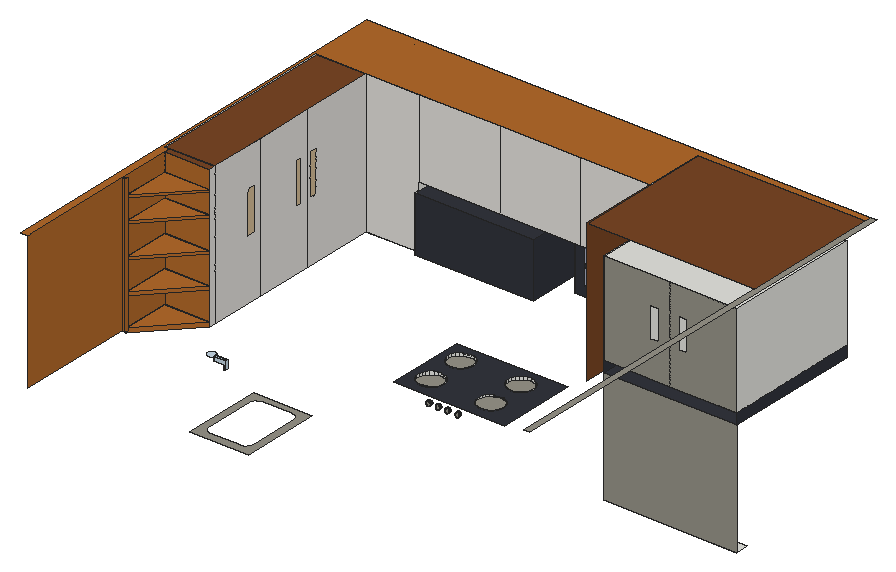
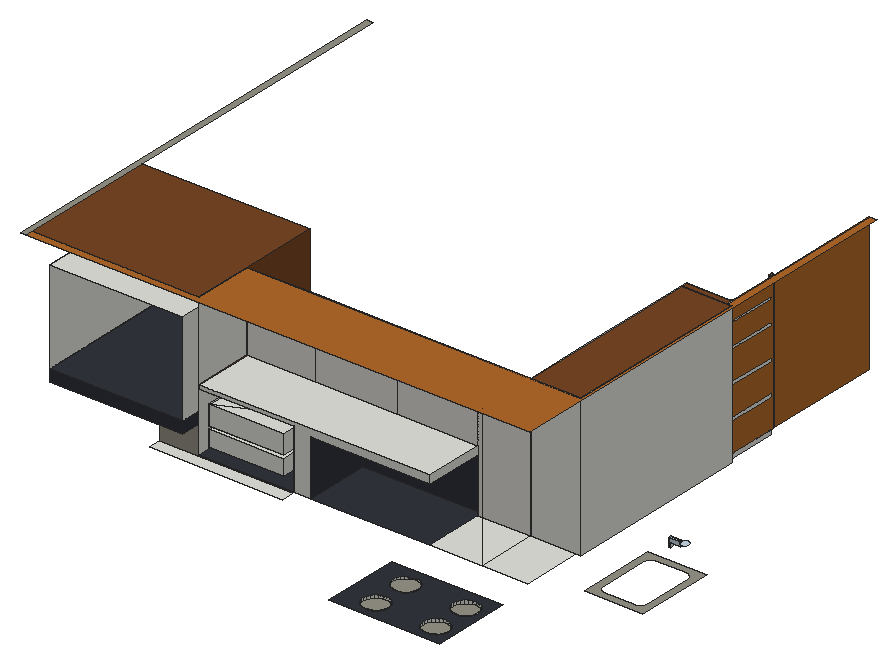
# SketchUp Ruby script. Lengths in inches.
U = 1.inch
M = Sketchup.active_model
def pt(a) = Geom::Point3d.new(a.map { |v| v * U })
def face(e, loops, mat)
  f = e.add_face(loops[0].map { |a| pt(a) })
  loops[1..].each { |l| e.add_face(l.map { |a| pt(a) }).erase! }
  f.material = f.back_material = mat if mat
  f
end
# faces: each face lists its corners as indices into pts; further lists are holes
def faces(e, pts, list, mat = nil) = list.each { |f| face(e, (f[0].is_a?(Array) ? f : [f]).map { |l| l.map { |i| pts[i] } }, mat) }
# xy, xz, yz: faces in a plane at the given z, y or x. An outline is a flat list of corners, or four numbers for a rectangle; further outlines are holes
def ring(l) = l.size == 4 ? [[l[0], l[1]], [l[2], l[1]], [l[2], l[3]], [l[0], l[3]]] : l.each_slice(2).to_a
def flat(e, list, mat, &to3) = list.each { |f| face(e, (f[0].is_a?(Array) ? f : [f]).map { |l| ring(l).map { |u, v| to3.(u, v) } }, mat) }
def xy(e, z, list, mat = nil) = flat(e, list, mat) { |x, y| [x, y, z] }
def xz(e, y, list, mat = nil) = flat(e, list, mat) { |x, z| [x, y, z] }
def yz(e, x, list, mat = nil) = flat(e, list, mat) { |y, z| [x, y, z] }
def lines(e, pts, list) = list.each { |a, b| e.add_line(pt(pts[a]), pt(pts[b])) }
# prism: a flat outline (further loops are holes) pulled along v
def prism(e, loops, v, mat = nil)
  f = face(e, loops, mat); d = Geom::Vector3d.new(v.map { |x| x * U })
  f.pushpull(f.normal.samedirection?(d) ? d.length : -d.length)
end
def box(e, o, s, mat = nil) = prism(e, [[o, [o[0] + s[0], o[1], o[2]], [o[0] + s[0], o[1] + s[1], o[2]], [o[0], o[1] + s[1], o[2]]]], [0, 0, s[2]], mat)
def at(x, y, z, deg = 0) = Geom::Transformation.translation(pt([x, y, z])) * Geom::Transformation.rotation(ORIGIN, Z_AXIS, deg.degrees)
def axes(o, x, y, z) = Geom::Transformation.new([*x, 0, *y, 0, *z, 0, *pt(o).to_a, 1])
def part(name) = M.definitions.add(name)
# library, detail: a bought-in or finely detailed component or shape, given as its bounding box
def library(name, o, s) = part(name).tap { |d| box(d.entities, o, s) }
def detail(e, o, s) = box(e.add_group.entities, o, s)
def put(e, d, t, mat = nil) = e.add_instance(d, t).tap { |i| i.material = mat if mat }
def group(e, t, mat = nil) = e.add_group.tap { |g| g.transformation = t; g.material = mat if mat }.entities
root = M.entities
M.materials.add("[Formica Beige]").color = [211, 187, 149]
M.materials.add("[Formica Graystone]").color = [149, 146, 135]
M.materials.add("[Formica Laminate Dark]").color = [50, 53, 60]
M.materials.add("[Terrazzo Light Blue]").color = [196, 214, 227]
M.materials.add("[Terrazzo Tile Accent]").color = [224, 221, 217]
M.materials.add("[Translucent Glass Sky Reflection]").color = [126, 138, 183]
M.materials["[Translucent Glass Sky Reflection]"].alpha = 0.52
M.materials.add("[Wood Bamboo]").color = [177, 105, 43]
M.materials.add("[Wood Veneer 01]").color = [120, 70, 37]
xy(root,44.875,[[[7.92,55.33,25.99,79.71],[12.63,57.43,12.29,57.45,11.96,57.52,11.63,57.625,11.33,57.78,11.04,57.97,10.78,58.19,10.56,58.45,10.37,58.73,10.22,59.04,10.11,59.36,10.04,59.7,10.02,60.04,10.02,75.53,10.04,75.8,10.09,76.07,10.18,76.33,10.3,76.57,10.45,76.8,10.63,77,10.84,77.18,11.0625,77.33,11.31,77.45,11.57,77.54,11.83,77.6,12.11,77.61,21.58,77.61,21.89,77.59,22.18,77.53,22.47,77.4375,22.74,77.3,22.99,77.14,23.22,76.9375,23.42,76.71,23.58,76.46,23.72,76.1875,23.8125,75.9,23.87,75.61,23.89,75.31,23.89,59.85,23.87,59.54,23.81,59.23,23.71,58.93,23.57,58.64,23.39,58.375,23.18,58.14,22.94,57.93,22.68,57.75,22.39,57.61,22.09,57.51,21.78,57.45,21.47,57.43]]],"[Formica Graystone]")
xy(root,46.625,[[40.04,104,41.05,104.13,41.98,104.52,42.78,105.13,43.4,105.93,43.79,106.87,43.92,107.87,43.79,108.875,43.4,109.81,42.78,110.61,41.98,111.23,41.05,111.61,40.04,111.75,39.04,111.61,38.11,111.23,37.3,110.61,36.6875,109.81,36.3,108.875,36.17,107.87,36.3,106.87,36.6875,105.93,37.3,105.13,38.11,104.52,39.04,104.13]],"[Formica Graystone]")
xy(root,46.64,[[108.5,88.5625,149.5,92.5]])
xy(root,46.6875,[[39.92,115.43,40.92,115.57,41.86,115.95,42.66,116.57,43.27,117.37,43.66,118.31,43.79,119.31,43.66,120.3125,43.27,121.25,42.66,122.05,41.86,122.66,40.92,123.05,39.92,123.18,38.92,123.05,37.98,122.66,37.18,122.05,36.5625,121.25,36.17,120.3125,36.04,119.31,36.17,118.31,36.5625,117.37,37.18,116.57,37.98,115.95,38.92,115.57],[58.48,115.43,59.48,115.57,60.42,115.95,61.22,116.57,61.84,117.37,62.22,118.31,62.36,119.31,62.22,120.3125,61.84,121.25,61.22,122.05,60.42,122.66,59.48,123.05,58.48,123.18,57.48,123.05,56.54,122.66,55.74,122.05,55.125,121.25,54.74,120.3125,54.61,119.31,54.74,118.31,55.125,117.37,55.74,116.57,56.54,115.95,57.48,115.57]],"[Formica Graystone]")
xy(root,47.0625,[[58.48,104,59.48,104.13,60.42,104.52,61.22,105.13,61.84,105.93,62.22,106.87,62.36,107.87,62.22,108.875,61.84,109.81,61.22,110.61,60.42,111.23,59.48,111.61,58.48,111.75,57.48,111.61,56.54,111.23,55.74,110.61,55.125,109.81,54.74,108.875,54.61,107.87,54.74,106.87,55.125,105.93,55.74,105.13,56.54,104.52,57.48,104.13]],"[Formica Graystone]")
xy(root,47.5,[[[34.11,101.1,68.05,125.35],[39.92,115.43,38.92,115.57,37.98,115.95,37.18,116.57,36.5625,117.37,36.17,118.31,36.04,119.31,36.17,120.3125,36.5625,121.25,37.18,122.05,37.98,122.66,38.92,123.05,39.92,123.18,40.92,123.05,41.86,122.66,42.66,122.05,43.27,121.25,43.66,120.3125,43.79,119.31,43.66,118.31,43.27,117.37,42.66,116.57,41.86,115.95,40.92,115.57],[58.48,115.43,57.48,115.57,56.54,115.95,55.74,116.57,55.125,117.37,54.74,118.31,54.61,119.31,54.74,120.3125,55.125,121.25,55.74,122.05,56.54,122.66,57.48,123.05,58.48,123.18,59.48,123.05,60.42,122.66,61.22,122.05,61.84,121.25,62.22,120.3125,62.36,119.31,62.22,118.31,61.84,117.37,61.22,116.57,60.42,115.95,59.48,115.57],[58.48,104,57.48,104.13,56.54,104.52,55.74,105.13,55.125,105.93,54.74,106.87,54.61,107.87,54.74,108.875,55.125,109.81,55.74,110.61,56.54,111.23,57.48,111.61,58.48,111.75,59.48,111.61,60.42,111.23,61.22,110.61,61.84,109.81,62.22,108.875,62.36,107.87,62.22,106.87,61.84,105.93,61.22,105.13,60.42,104.52,59.48,104.13],[40.04,104,39.04,104.13,38.11,104.52,37.3,105.13,36.6875,105.93,36.3,106.87,36.17,107.87,36.3,108.875,36.6875,109.81,37.3,110.61,38.11,111.23,39.04,111.61,40.04,111.75,41.05,111.61,41.98,111.23,42.78,110.61,43.4,109.81,43.79,108.875,43.92,107.87,43.79,106.87,43.4,105.93,42.78,105.13,41.98,104.52,41.05,104.13]]],"[Formica Laminate Dark]")
xy(root,57.375,[[9.09,66.7,9.81,67.6]])
xy(root,58.5625,[[6.04,66.7,6.16,66.99,6.2,67.29,6.16,67.6,9.09,67.6,9.09,66.7]])
xy(root,59.875,[[6.04,66.7,6.16,66.99,6.2,67.29,6.16,67.6,6.04,67.6]])
xy(root,59.875,[[5.01,66.11,5.32,66.15,5.61,66.27,5.85,66.45,6.04,66.7,6.04,67.6,6.16,67.6,6.04,67.89,5.85,68.13,5.61,68.32,5.32,68.44,5.01,68.48,4.71,68.44,4.42,68.32,4.17,68.13,3.99,67.89,3.87,67.6,3.83,67.29,3.87,66.99,3.99,66.7,4.17,66.45,4.42,66.27,4.71,66.15],[6.04,66.7,9.81,66.7,9.81,67.6,6.16,67.6,6.2,67.29,6.16,66.99]],"[Terrazzo Light Blue]")
xy(root,77.75,[[0.9375,54.54,2.25,112.625],[2.25,112.625,16.25,131.0625],[16.25,112.625,32.46,131.0625]])
xy(root,77.75,[[32.46,111.0625,68.96,131.0625],[74.1875,120.3125,103.5,131.0625]],"[Formica Laminate Dark]")
xy(root,77.75,[[2.25,37.75,2.25,52.57,16.25,52.57],[2.25,52.57,16.25,54.54],[2.25,54.54,16.25,112.625]],"[Wood Bamboo]")
xy(root,79.12,[[2.25,36.1,3.375,36.93],[2.25,37.75,16.25,52.57,2.25,52.57]],"[Wood Bamboo]")
xy(root,80.93,[[77.37,120.3125,100.32,131.0625]])
xy(root,81.6875,[[108.5,88.5625,149.5,131.0625]],"[Formica Laminate Dark]")
xy(root,85.21,[[108.5,88.5625,149.5,131.0625]],"[Formica Laminate Dark]")
xy(root,85.84,[[77.37,120.3125,100.32,131.0625]])
xy(root,86.81,[[77.37,120.3125,100.32,131.0625]])
xy(root,88,[[2.25,37.75,2.25,52.57,16.25,52.57]],"[Wood Bamboo]")
xy(root,89.06,[[2.25,37.75,16.25,52.57,2.25,52.57]],"[Wood Bamboo]")
xy(root,92.68,[[77.37,120.3125,100.32,131.0625,100.32,120.3125],[77.37,120.3125,77.37,131.0625,100.32,131.0625]])
xy(root,94.62,[[32.46,111.0625,68.96,131.0625]],"[Formica Laminate Dark]")
xy(root,95.86,[[74.1875,120.3125,103.5,131.0625]])
xy(root,96.97,[[32.46,112.625,103.5,131.0625]])
xy(root,97.9,[[2.25,37.75,2.25,52.57,16.25,52.57]],"[Wood Bamboo]")
xy(root,98.72,[[2.25,37.75,16.25,52.57,2.25,52.57]],"[Wood Bamboo]")
xy(root,107.81,[[2.25,37.75,2.25,52.57,16.25,52.57]],"[Wood Bamboo]")
xy(root,108.56,[[2.25,37.75,16.25,52.57,2.25,52.57]],"[Wood Bamboo]")
xy(root,113.88,[[108.5,88.5625,149.5,131.0625]])
xy(root,115,[[2.25,37.75,2.25,52.57,16.25,52.57]],"[Wood Bamboo]")
xy(root,115.68,[[2.25,37.75,16.25,52.57,2.25,52.57]],"[Wood Bamboo]")
xy(root,121.1875,[[154.9375,0,156.6875,133.25]],"[Formica Graystone]")
xy(root,121.1875,[[0,0,2.25,0,2.25,36.1,3.375,36.1,3.375,36.93,2.25,36.93,2.25,54.54,0.9375,54.54,0.9375,112.625,103.5,112.625,103.5,131.0625,154.9375,131.0625,154.9375,133.25,0,133.25]],"[Wood Bamboo]")
xy(root,121.1875,[[2.25,52.57,16.25,54.54],[0.9375,54.54,16.25,112.625],[103.5,88.5625,154.9375,131.0625]],"[Wood Veneer 01]")
xz(root,36.1,[[2.25,79.12,3.375,121.1875]],"[Wood Bamboo]")
xz(root,36.93,[[2.25,79.12,3.375,121.1875]],"[Wood Bamboo]")
xz(root,52.57,[[2.25,77.75,16.25,79.12],[2.25,88,16.25,89.06],[2.25,97.9,16.25,98.72],[2.25,107.81,16.25,108.56],[2.25,115,16.25,115.68]])
xz(root,52.57,[[2.25,79.12,16.25,88],[2.25,89.06,16.25,97.9],[2.25,98.72,16.25,107.81],[2.25,108.56,16.25,115],[2.25,115.68,16.25,121.1875]],"[Wood Bamboo]")
xz(root,54.54,[[0.9375,77.75,2.25,121.1875],[2.25,77.75,16.25,121.1875]])
xz(root,66.7,[[9.09,57.375,9.81,57.375,9.81,59.875,6.04,59.875,6.04,58.5625,9.09,58.5625]],"[Terrazzo Light Blue]")
xz(root,67.6,[[9.09,57.375,9.09,58.5625,6.16,58.5625,6.16,59.875,9.81,59.875,9.81,57.375]],"[Terrazzo Light Blue]")
xz(root,88.5625,[[123.23,96.37,125.23,105.31],[131.86,96.37,133.86,105.31]])
xz(root,88.5625,[[108.5,46.64,149.5,81.6875],[[108.5,85.21,129,113.88],[123.23,96.37,125.23,105.31]],[[129,85.21,149.5,113.88],[131.86,96.37,133.86,105.31]]],"[Formica Graystone]")
xz(root,100.41,[[45.19,45.12,45.37,45.14,45.54,45.21,45.68,45.32,45.79,45.46,45.86,45.625,45.88,45.8,45.86,45.98,45.79,46.15,45.68,46.29,45.54,46.4,45.37,46.47,45.19,46.49,45.02,46.47,44.85,46.4,44.71,46.29,44.6,46.15,44.53,45.98,44.51,45.8,44.53,45.625,44.6,45.46,44.71,45.32,44.85,45.21,45.02,45.14],[48.01,45.12,48.18,45.14,48.35,45.21,48.49,45.32,48.6,45.46,48.67,45.625,48.69,45.8,48.67,45.98,48.6,46.15,48.49,46.29,48.35,46.4,48.18,46.47,48.01,46.49,47.83,46.47,47.66,46.4,47.52,46.29,47.41,46.15,47.34,45.98,47.32,45.8,47.34,45.625,47.41,45.46,47.52,45.32,47.66,45.21,47.83,45.14],[50.88,45.12,51.06,45.14,51.22,45.21,51.37,45.32,51.48,45.46,51.55,45.625,51.57,45.8,51.55,45.98,51.48,46.15,51.37,46.29,51.22,46.4,51.06,46.47,50.88,46.49,50.7,46.47,50.54,46.4,50.39,46.29,50.29,46.15,50.22,45.98,50.19,45.8,50.22,45.625,50.29,45.46,50.39,45.32,50.54,45.21,50.7,45.14],[54.07,45.12,54.25,45.14,54.41,45.21,54.55,45.32,54.66,45.46,54.73,45.625,54.76,45.8,54.73,45.98,54.66,46.15,54.55,46.29,54.41,46.4,54.25,46.47,54.07,46.49,53.89,46.47,53.72,46.4,53.58,46.29,53.47,46.15,53.4,45.98,53.38,45.8,53.4,45.625,53.47,45.46,53.58,45.32,53.72,45.21,53.89,45.14]],"[Formica Graystone]")
xz(root,101.1,[[45.19,45.12,45.02,45.14,44.85,45.21,44.71,45.32,44.6,45.46,44.53,45.625,44.51,45.8,44.53,45.98,44.6,46.15,44.71,46.29,44.85,46.4,45.02,46.47,45.19,46.49,45.37,46.47,45.54,46.4,45.68,46.29,45.79,46.15,45.86,45.98,45.88,45.8,45.86,45.625,45.79,45.46,45.68,45.32,45.54,45.21,45.37,45.14],[48.01,45.12,47.83,45.14,47.66,45.21,47.52,45.32,47.41,45.46,47.34,45.625,47.32,45.8,47.34,45.98,47.41,46.15,47.52,46.29,47.66,46.4,47.83,46.47,48.01,46.49,48.18,46.47,48.35,46.4,48.49,46.29,48.6,46.15,48.67,45.98,48.69,45.8,48.67,45.625,48.6,45.46,48.49,45.32,48.35,45.21,48.18,45.14],[50.88,45.12,50.7,45.14,50.54,45.21,50.39,45.32,50.29,45.46,50.22,45.625,50.19,45.8,50.22,45.98,50.29,46.15,50.39,46.29,50.54,46.4,50.7,46.47,50.88,46.49,51.06,46.47,51.22,46.4,51.37,46.29,51.48,46.15,51.55,45.98,51.57,45.8,51.55,45.625,51.48,45.46,51.37,45.32,51.22,45.21,51.06,45.14],[54.07,45.12,53.89,45.14,53.72,45.21,53.58,45.32,53.47,45.46,53.4,45.625,53.38,45.8,53.4,45.98,53.47,46.15,53.58,46.29,53.72,46.4,53.89,46.47,54.07,46.49,54.25,46.47,54.41,46.4,54.55,46.29,54.66,46.15,54.73,45.98,54.76,45.8,54.73,45.625,54.66,45.46,54.55,45.32,54.41,45.21,54.25,45.14]])
xz(root,111.0625,[[32.46,77.75,68.96,94.62]],"[Formica Laminate Dark]")
xz(root,112.625,[[0.9375,77.75,16.25,121.1875]])
xz(root,112.625,[[16.25,77.75,32.46,121.1875],[32.46,96.97,57.4375,121.1875],[57.4375,96.97,82.42,121.1875],[82.42,96.97,103.5,121.1875]],"[Terrazzo Tile Accent]")
xz(root,120.3125,[[[74.1875,77.75,103.5,95.86],[77.37,80.93,100.32,92.68]],[77.37,85.84,100.32,86.81]],"[Formica Laminate Dark]")
xz(root,120.3125,[[77.37,80.93,100.32,85.84],[77.37,86.81,100.32,92.68]],"[Translucent Glass Sky Reflection]")
xz(root,131.0625,[[68.96,77.75,74.1875,77.75,74.1875,95.86,103.5,95.86,103.5,96.97,32.46,96.97,32.46,94.62,68.96,94.62],[77.37,80.93,100.32,85.84],[77.37,86.81,100.32,92.68]])
xz(root,131.0625,[[108.5,81.6875,149.5,85.21]],"[Formica Laminate Dark]")
yz(root,0.9375,[[54.54,77.75,112.625,121.1875]])
yz(root,2.25,[[37.75,77.75,52.57,79.12],[52.57,77.75,54.54,121.1875],[37.75,88,52.57,89.06],[37.75,97.9,52.57,98.72],[37.75,107.81,52.57,108.56],
  [37.75,115,52.57,115.68]])
yz(root,2.25,[[0,79.12,36.1,121.1875],[36.93,79.12,52.57,79.12,52.57,88,37.75,88,37.75,89.06,52.57,89.06,52.57,97.9,37.75,97.9,37.75,98.72,52.57,98.72,52.57,107.81,37.75,107.81,37.75,108.56,52.57,108.56,52.57,115,37.75,115,37.75,115.68,52.57,115.68,52.57,121.1875,36.93,121.1875]],"[Wood Bamboo]")
yz(root,3.375,[[36.1,79.12,36.93,121.1875]],"[Wood Bamboo]")
yz(root,9.09,[[66.7,57.375,67.6,58.5625]])
yz(root,9.81,[[66.7,57.375,67.6,59.875]],"[Terrazzo Light Blue]")
yz(root,16.25,[[67.33,96.42,69.52,109.23],[85.52,96.42,87.71,109.23],[91.15,96.42,93.33,109.23]],"[Formica Beige]")
yz(root,16.25,[[52.57,77.75,54.54,121.1875],[[54.54,77.75,71.97,121.1875],[67.33,96.42,69.52,109.23]],[[71.97,77.75,89.83,121.1875],[85.52,96.42,87.71,109.23]],[[89.83,77.75,112.625,121.1875],[91.15,96.42,93.33,109.23]]],"[Terrazzo Tile Accent]")
yz(root,32.46,[[111.0625,77.75,112.625,94.62],[112.625,94.62,131.0625,96.97]])
yz(root,68.96,[[111.0625,77.75,131.0625,94.62]],"[Formica Laminate Dark]")
yz(root,74.1875,[[120.3125,77.75,131.0625,95.86]],"[Formica Laminate Dark]")
yz(root,77.37,[[120.3125,80.93,131.0625,85.84],[120.3125,86.81,131.0625,92.68]])
yz(root,100.32,[[120.3125,80.93,131.0625,85.84],[120.3125,86.81,131.0625,92.68]])
yz(root,103.5,[[120.3125,77.75,131.0625,95.86],[112.625,96.97,131.0625,121.1875]])
yz(root,103.5,[[88.5625,77.75,88.5625,121.1875,112.625,121.1875,112.625,96.97,131.0625,96.97,131.0625,95.86,120.3125,95.86,120.3125,77.75]],"[Wood Veneer 01]")
yz(root,108.5,[[88.5625,85.21,131.0625,113.88]])
yz(root,108.5,[[88.5625,81.6875,131.0625,85.21]],"[Formica Laminate Dark]")
yz(root,149.5,[[88.5625,85.21,131.0625,113.88]])
yz(root,149.5,[[88.5625,81.6875,131.0625,85.21]],"[Formica Laminate Dark]")
p = [[44.85,101.1,45.21],[45.02,101.1,45.14],[45.02,100.41,45.14],[44.85,100.41,45.21],[45.19,101.1,45.12],[45.19,100.41,45.12],
  [45.37,101.1,45.14],[45.37,100.41,45.14],[45.54,101.1,45.21],[45.54,100.41,45.21],[47.66,101.1,45.21],[47.83,101.1,45.14],
  [47.83,100.41,45.14],[47.66,100.41,45.21],[48.01,101.1,45.12],[48.01,100.41,45.12],[48.18,101.1,45.14],[48.18,100.41,45.14],
  [48.35,101.1,45.21],[48.35,100.41,45.21],[50.54,101.1,45.21],[50.7,101.1,45.14],[50.7,100.41,45.14],[50.54,100.41,45.21],
  [50.88,101.1,45.12],[50.88,100.41,45.12],[51.06,101.1,45.14],[51.06,100.41,45.14],[51.22,101.1,45.21],[51.22,100.41,45.21],
  [53.72,101.1,45.21],[53.89,101.1,45.14],[53.89,100.41,45.14],[53.72,100.41,45.21],[54.07,101.1,45.12],[54.07,100.41,45.12],
  [54.25,101.1,45.14],[54.25,100.41,45.14],[54.41,101.1,45.21],[54.41,100.41,45.21],[44.71,101.1,45.32],[44.71,100.41,45.32],
  [45.68,101.1,45.32],[45.68,100.41,45.32],[47.52,101.1,45.32],[47.52,100.41,45.32],[48.49,101.1,45.32],[48.49,100.41,45.32],
  [50.39,101.1,45.32],[50.39,100.41,45.32],[51.37,101.1,45.32],[51.37,100.41,45.32],[53.58,101.1,45.32],[53.58,100.41,45.32],
  [54.55,101.1,45.32],[54.55,100.41,45.32],[44.6,101.1,45.46],[44.6,100.41,45.46],[45.79,101.1,45.46],[45.79,100.41,45.46],
  [47.41,101.1,45.46],[47.41,100.41,45.46],[48.6,101.1,45.46],[48.6,100.41,45.46],[50.29,101.1,45.46],[50.29,100.41,45.46],
  [51.48,101.1,45.46],[51.48,100.41,45.46],[53.47,101.1,45.46],[53.47,100.41,45.46],[54.66,101.1,45.46],[54.66,100.41,45.46],
  [44.53,101.1,45.625],[44.53,100.41,45.625],[45.86,101.1,45.625],[45.86,100.41,45.625],[47.34,101.1,45.625],[47.34,100.41,45.625],
  [48.67,101.1,45.625],[48.67,100.41,45.625],[50.22,101.1,45.625],[50.22,100.41,45.625],[51.55,101.1,45.625],[51.55,100.41,45.625],
  [53.4,101.1,45.625],[53.4,100.41,45.625],[54.73,101.1,45.625],[54.73,100.41,45.625],[44.51,101.1,45.8],[44.51,100.41,45.8],
  [45.88,101.1,45.8],[45.88,100.41,45.8],[47.32,101.1,45.8],[47.32,100.41,45.8],[48.69,101.1,45.8],[48.69,100.41,45.8],
  [50.19,101.1,45.8],[50.19,100.41,45.8],[51.57,101.1,45.8],[51.57,100.41,45.8],[53.38,101.1,45.8],[53.38,100.41,45.8],
  [54.76,101.1,45.8],[54.76,100.41,45.8],[44.53,101.1,45.98],[44.53,100.41,45.98],[45.86,101.1,45.98],[45.86,100.41,45.98],
  [47.34,101.1,45.98],[47.34,100.41,45.98],[48.67,101.1,45.98],[48.67,100.41,45.98],[50.22,101.1,45.98],[50.22,100.41,45.98],
  [51.55,101.1,45.98],[51.55,100.41,45.98],[53.4,101.1,45.98],[53.4,100.41,45.98],[54.73,101.1,45.98],[54.73,100.41,45.98],
  [44.6,101.1,46.15],[44.6,100.41,46.15],[45.79,101.1,46.15],[45.79,100.41,46.15],[47.41,101.1,46.15],[47.41,100.41,46.15],
  [48.6,101.1,46.15],[48.6,100.41,46.15],[50.29,101.1,46.15],[50.29,100.41,46.15],[51.48,101.1,46.15],[51.48,100.41,46.15],
  [53.47,101.1,46.15],[53.47,100.41,46.15],[54.66,101.1,46.15],[54.66,100.41,46.15],[44.71,101.1,46.29],[44.71,100.41,46.29],
  [45.68,101.1,46.29],[45.68,100.41,46.29],[47.52,101.1,46.29],[47.52,100.41,46.29],[48.49,101.1,46.29],[48.49,100.41,46.29],
  [50.39,101.1,46.29],[50.39,100.41,46.29],[51.37,101.1,46.29],[51.37,100.41,46.29],[53.58,101.1,46.29],[53.58,100.41,46.29],
  [54.55,101.1,46.29],[54.55,100.41,46.29],[44.85,101.1,46.4],[44.85,100.41,46.4],[45.54,101.1,46.4],[45.54,100.41,46.4],
  [47.66,101.1,46.4],[47.66,100.41,46.4],[48.35,101.1,46.4],[48.35,100.41,46.4],[50.54,101.1,46.4],[50.54,100.41,46.4],
  [51.22,101.1,46.4],[51.22,100.41,46.4],[53.72,101.1,46.4],[53.72,100.41,46.4],[54.41,101.1,46.4],[54.41,100.41,46.4],
  [45.02,101.1,46.47],[45.02,100.41,46.47],[45.37,101.1,46.47],[45.37,100.41,46.47],[47.83,101.1,46.47],[47.83,100.41,46.47],
  [48.18,101.1,46.47],[48.18,100.41,46.47],[50.7,101.1,46.47],[50.7,100.41,46.47],[51.06,101.1,46.47],[51.06,100.41,46.47],
  [53.89,101.1,46.47],[53.89,100.41,46.47],[54.25,101.1,46.47],[54.25,100.41,46.47],[45.19,101.1,46.49],[45.19,100.41,46.49],
  [48.01,101.1,46.49],[48.01,100.41,46.49],[50.88,101.1,46.49],[50.88,100.41,46.49],[54.07,101.1,46.49],[54.07,100.41,46.49],
  [39.04,104.13,47.5],[40.04,104,47.5],[40.04,104,46.625],[39.04,104.13,46.625],[41.05,104.13,47.5],[41.05,104.13,46.625],
  [38.11,104.52,47.5],[38.11,104.52,46.625],[41.98,104.52,47.5],[41.98,104.52,46.625],[37.3,105.13,47.5],[37.3,105.13,46.625],
  [42.78,105.13,47.5],[42.78,105.13,46.625],[36.6875,105.93,47.5],[36.6875,105.93,46.625],[43.4,105.93,47.5],[43.4,105.93,46.625],
  [36.3,106.87,47.5],[36.3,106.87,46.625],[43.79,106.87,47.5],[43.79,106.87,46.625],[36.17,107.87,47.5],[36.17,107.87,46.625],
  [43.92,107.87,47.5],[43.92,107.87,46.625],[36.3,108.875,47.5],[36.3,108.875,46.625],[43.79,108.875,47.5],[43.79,108.875,46.625],
  [36.6875,109.81,47.5],[36.6875,109.81,46.625],[43.4,109.81,47.5],[43.4,109.81,46.625],[37.3,110.61,47.5],[37.3,110.61,46.625],
  [42.78,110.61,47.5],[42.78,110.61,46.625],[38.11,111.23,47.5],[38.11,111.23,46.625],[41.98,111.23,47.5],[41.98,111.23,46.625],
  [39.04,111.61,47.5],[39.04,111.61,46.625],[41.05,111.61,47.5],[41.05,111.61,46.625],[40.04,111.75,47.5],[40.04,111.75,46.625],
  [38.92,115.57,47.5],[39.92,115.43,47.5],[39.92,115.43,46.6875],[38.92,115.57,46.6875],[40.92,115.57,47.5],[40.92,115.57,46.6875],
  [57.48,115.57,47.5],[58.48,115.43,47.5],[58.48,115.43,46.6875],[57.48,115.57,46.6875],[59.48,115.57,47.5],[59.48,115.57,46.6875],
  [37.98,115.95,47.5],[37.98,115.95,46.6875],[41.86,115.95,47.5],[41.86,115.95,46.6875],[56.54,115.95,47.5],[56.54,115.95,46.6875],
  [60.42,115.95,47.5],[60.42,115.95,46.6875],[37.18,116.57,47.5],[37.18,116.57,46.6875],[42.66,116.57,47.5],[42.66,116.57,46.6875],
  [55.74,116.57,47.5],[55.74,116.57,46.6875],[61.22,116.57,47.5],[61.22,116.57,46.6875],[36.5625,117.37,47.5],[36.5625,117.37,46.6875],
  [43.27,117.37,47.5],[43.27,117.37,46.6875],[55.125,117.37,47.5],[55.125,117.37,46.6875],[61.84,117.37,47.5],[61.84,117.37,46.6875],
  [36.17,118.31,47.5],[36.17,118.31,46.6875],[43.66,118.31,47.5],[43.66,118.31,46.6875],[54.74,118.31,47.5],[54.74,118.31,46.6875],
  [62.22,118.31,47.5],[62.22,118.31,46.6875],[36.04,119.31,47.5],[36.04,119.31,46.6875],[43.79,119.31,47.5],[43.79,119.31,46.6875],
  [54.61,119.31,47.5],[54.61,119.31,46.6875],[62.36,119.31,47.5],[62.36,119.31,46.6875],[36.17,120.3125,47.5],[36.17,120.3125,46.6875],
  [43.66,120.3125,47.5],[43.66,120.3125,46.6875],[54.74,120.3125,47.5],[54.74,120.3125,46.6875],[62.22,120.3125,47.5],[62.22,120.3125,46.6875],
  [36.5625,121.25,47.5],[36.5625,121.25,46.6875],[43.27,121.25,47.5],[43.27,121.25,46.6875],[55.125,121.25,47.5],[55.125,121.25,46.6875],
  [61.84,121.25,47.5],[61.84,121.25,46.6875],[37.18,122.05,47.5],[37.18,122.05,46.6875],[42.66,122.05,47.5],[42.66,122.05,46.6875],
  [55.74,122.05,47.5],[55.74,122.05,46.6875],[61.22,122.05,47.5],[61.22,122.05,46.6875],[37.98,122.66,47.5],[37.98,122.66,46.6875],
  [41.86,122.66,47.5],[41.86,122.66,46.6875],[56.54,122.66,47.5],[56.54,122.66,46.6875],[60.42,122.66,47.5],[60.42,122.66,46.6875],
  [38.92,123.05,47.5],[38.92,123.05,46.6875],[40.92,123.05,47.5],[40.92,123.05,46.6875],[57.48,123.05,47.5],[57.48,123.05,46.6875],
  [59.48,123.05,47.5],[59.48,123.05,46.6875],[39.92,123.18,47.5],[39.92,123.18,46.6875],[58.48,123.18,47.5],[58.48,123.18,46.6875],
  [57.48,104.13,47.5],[58.48,104,47.5],[58.48,104,47.0625],[57.48,104.13,47.0625],[59.48,104.13,47.5],[59.48,104.13,47.0625],
  [56.54,104.52,47.5],[56.54,104.52,47.0625],[60.42,104.52,47.5],[60.42,104.52,47.0625],[55.74,105.13,47.5],[55.74,105.13,47.0625],
  [61.22,105.13,47.5],[61.22,105.13,47.0625],[55.125,105.93,47.5],[55.125,105.93,47.0625],[61.84,105.93,47.5],[61.84,105.93,47.0625],
  [54.74,106.87,47.5],[54.74,106.87,47.0625],[62.22,106.87,47.5],[62.22,106.87,47.0625],[54.61,107.87,47.5],[54.61,107.87,47.0625],
  [62.36,107.87,47.5],[62.36,107.87,47.0625],[54.74,108.875,47.5],[54.74,108.875,47.0625],[62.22,108.875,47.5],[62.22,108.875,47.0625],
  [55.125,109.81,47.5],[55.125,109.81,47.0625],[61.84,109.81,47.5],[61.84,109.81,47.0625],[55.74,110.61,47.5],[55.74,110.61,47.0625],
  [61.22,110.61,47.5],[61.22,110.61,47.0625],[56.54,111.23,47.5],[56.54,111.23,47.0625],[60.42,111.23,47.5],[60.42,111.23,47.0625],
  [57.48,111.61,47.5],[57.48,111.61,47.0625],[59.48,111.61,47.5],[59.48,111.61,47.0625],[58.48,111.75,47.5],[58.48,111.75,47.0625],
  [6.16,66.99,59.875],[6.04,66.7,59.875],[6.04,66.7,58.5625],[6.16,66.99,58.5625],[6.2,67.29,59.875],[6.2,67.29,58.5625],
  [6.16,67.6,59.875],[6.16,67.6,58.5625],[2.25,37.75,77.75],[16.25,52.57,77.75],[16.25,52.57,79.12],[2.25,37.75,79.12],
  [2.25,37.75,88],[16.25,52.57,88],[16.25,52.57,89.06],[2.25,37.75,89.06],[2.25,37.75,97.9],[16.25,52.57,97.9],
  [16.25,52.57,98.72],[2.25,37.75,98.72],[2.25,37.75,107.81],[16.25,52.57,107.81],[16.25,52.57,108.56],[2.25,37.75,108.56],
  [2.25,37.75,115],[16.25,52.57,115],[16.25,52.57,115.68],[2.25,37.75,115.68],[16.25,131.0625,77.75],[16.25,131.0625,121.1875]]
faces(root,p,[[0,1,2,3],[1,4,5,2],[4,6,7,5],[6,8,9,7],[10,11,12,13],[11,14,15,12],[14,16,17,15],[16,18,19,17],
  [20,21,22,23],[21,24,25,22],[24,26,27,25],[26,28,29,27],[30,31,32,33],[31,34,35,32],[34,36,37,35],[36,38,39,37],
  [40,0,3,41],[8,42,43,9],[44,10,13,45],[18,46,47,19],[48,20,23,49],[28,50,51,29],[52,30,33,53],[38,54,55,39],
  [56,40,41,57],[42,58,59,43],[60,44,45,61],[46,62,63,47],[64,48,49,65],[50,66,67,51],[68,52,53,69],[54,70,71,55],
  [72,56,57,73],[58,74,75,59],[76,60,61,77],[62,78,79,63],[80,64,65,81],[66,82,83,67],[84,68,69,85],[70,86,87,71],
  [88,72,73,89],[74,90,91,75],[92,76,77,93],[78,94,95,79],[96,80,81,97],[82,98,99,83],[100,84,85,101],[86,102,103,87],
  [104,88,89,105],[90,106,107,91],[108,92,93,109],[94,110,111,95],[112,96,97,113],[98,114,115,99],[116,100,101,117],[102,118,119,103],
  [120,104,105,121],[106,122,123,107],[124,108,109,125],[110,126,127,111],[128,112,113,129],[114,130,131,115],[132,116,117,133],[118,134,135,119],
  [136,120,121,137],[122,138,139,123],[140,124,125,141],[126,142,143,127],[144,128,129,145],[130,146,147,131],[148,132,133,149],[134,150,151,135],
  [152,136,137,153],[138,154,155,139],[156,140,141,157],[142,158,159,143],[160,144,145,161],[146,162,163,147],[164,148,149,165],[150,166,167,151],
  [168,152,153,169],[154,170,171,155],[172,156,157,173],[158,174,175,159],[176,160,161,177],[162,178,179,163],[180,164,165,181],[166,182,183,167],
  [184,168,169,185],[170,184,185,171],[186,172,173,187],[174,186,187,175],[188,176,177,189],[178,188,189,179],[190,180,181,191],[182,190,191,183]],"[Formica Graystone]")
faces(root,p,[[192,193,194,195],[193,196,197,194],[198,192,195,199],[196,200,201,197],[202,198,199,203],[200,204,205,201],[206,202,203,207],[204,208,209,205],
  [210,206,207,211],[208,212,213,209],[214,210,211,215],[212,216,217,213],[218,214,215,219],[216,220,221,217],[222,218,219,223],[220,224,225,221],
  [226,222,223,227],[224,228,229,225],[230,226,227,231],[228,232,233,229],[234,230,231,235],[232,236,237,233],[238,234,235,239],[236,238,239,237],
  [240,241,242,243],[241,244,245,242],[246,247,248,249],[247,250,251,248],[252,240,243,253],[244,254,255,245],[256,246,249,257],[250,258,259,251],
  [260,252,253,261],[254,262,263,255],[264,256,257,265],[258,266,267,259],[268,260,261,269],[262,270,271,263],[272,264,265,273],[266,274,275,267],
  [276,268,269,277],[270,278,279,271],[280,272,273,281],[274,282,283,275],[284,276,277,285],[278,286,287,279],[288,280,281,289],[282,290,291,283],
  [292,284,285,293],[286,294,295,287],[296,288,289,297],[290,298,299,291],[300,292,293,301],[294,302,303,295],[304,296,297,305],[298,306,307,299],
  [308,300,301,309],[302,310,311,303],[312,304,305,313],[306,314,315,307],[316,308,309,317],[310,318,319,311],[320,312,313,321],[314,322,323,315],
  [324,316,317,325],[318,326,327,319],[328,320,321,329],[322,330,331,323],[332,324,325,333],[326,332,333,327],[334,328,329,335],[330,334,335,331],
  [336,337,338,339],[337,340,341,338],[342,336,339,343],[340,344,345,341],[346,342,343,347],[344,348,349,345],[350,346,347,351],[348,352,353,349],
  [354,350,351,355],[352,356,357,353],[358,354,355,359],[356,360,361,357],[362,358,359,363],[360,364,365,361],[366,362,363,367],[364,368,369,365],
  [370,366,367,371],[368,372,373,369],[374,370,371,375],[372,376,377,373],[378,374,375,379],[376,380,381,377],[382,378,379,383],[380,382,383,381],
  [384,385,386,387],[388,384,387,389],[390,388,389,391]])
faces(root,p,[[392,393,394,395],[396,397,398,399],[400,401,402,403],[404,405,406,407],[408,409,410,411]],"[Wood Bamboo]")
lines(root,p,[[412,413]])
